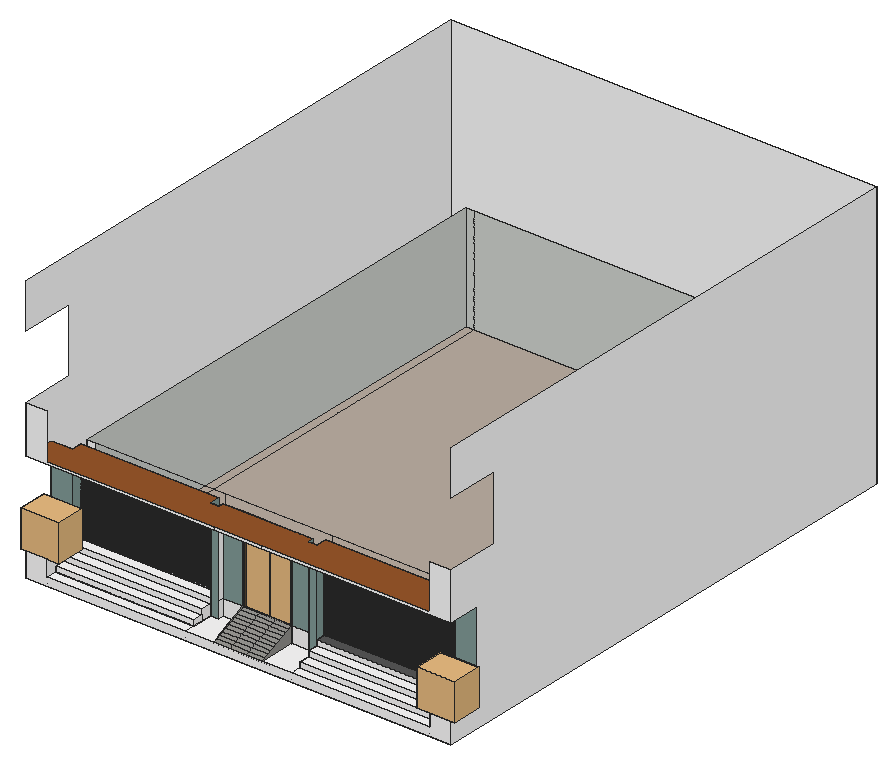
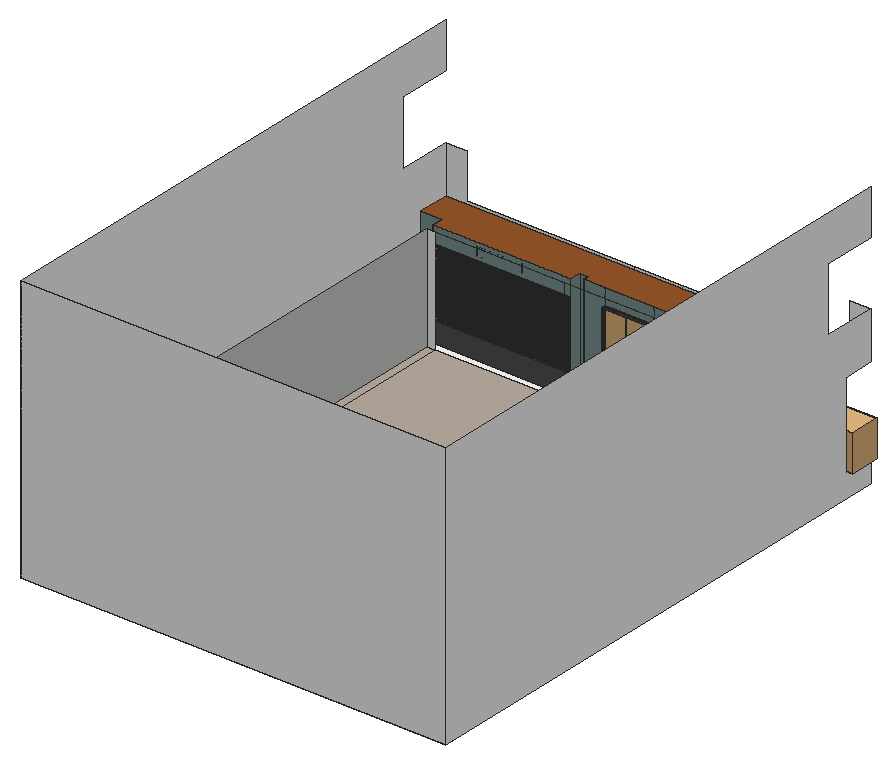
# SketchUp Ruby script. Lengths in inches.
U = 1.inch
M = Sketchup.active_model
def pt(a) = Geom::Point3d.new(a.map { |v| v * U })
def face(e, loops, mat)
  f = e.add_face(loops[0].map { |a| pt(a) })
  loops[1..].each { |l| e.add_face(l.map { |a| pt(a) }).erase! }
  f.material = f.back_material = mat if mat
  f
end
# faces: each face lists its corners as indices into pts; further lists are holes
def faces(e, pts, list, mat = nil) = list.each { |f| face(e, (f[0].is_a?(Array) ? f : [f]).map { |l| l.map { |i| pts[i] } }, mat) }
# xy, xz, yz: faces in a plane at the given z, y or x. An outline is a flat list of corners, or four numbers for a rectangle; further outlines are holes
def ring(l) = l.size == 4 ? [[l[0], l[1]], [l[2], l[1]], [l[2], l[3]], [l[0], l[3]]] : l.each_slice(2).to_a
def flat(e, list, mat, &to3) = list.each { |f| face(e, (f[0].is_a?(Array) ? f : [f]).map { |l| ring(l).map { |u, v| to3.(u, v) } }, mat) }
def xy(e, z, list, mat = nil) = flat(e, list, mat) { |x, y| [x, y, z] }
def xz(e, y, list, mat = nil) = flat(e, list, mat) { |x, z| [x, y, z] }
def yz(e, x, list, mat = nil) = flat(e, list, mat) { |y, z| [x, y, z] }
def lines(e, pts, list) = list.each { |a, b| e.add_line(pt(pts[a]), pt(pts[b])) }
# prism: a flat outline (further loops are holes) pulled along v
def prism(e, loops, v, mat = nil)
  f = face(e, loops, mat); d = Geom::Vector3d.new(v.map { |x| x * U })
  f.pushpull(f.normal.samedirection?(d) ? d.length : -d.length)
end
def box(e, o, s, mat = nil) = prism(e, [[o, [o[0] + s[0], o[1], o[2]], [o[0] + s[0], o[1] + s[1], o[2]], [o[0], o[1] + s[1], o[2]]]], [0, 0, s[2]], mat)
def at(x, y, z, deg = 0) = Geom::Transformation.translation(pt([x, y, z])) * Geom::Transformation.rotation(ORIGIN, Z_AXIS, deg.degrees)
def axes(o, x, y, z) = Geom::Transformation.new([*x, 0, *y, 0, *z, 0, *pt(o).to_a, 1])
def part(name) = M.definitions.add(name)
# library, detail: a bought-in or finely detailed component or shape, given as its bounding box
def library(name, o, s) = part(name).tap { |d| box(d.entities, o, s) }
def detail(e, o, s) = box(e.add_group.entities, o, s)
def put(e, d, t, mat = nil) = e.add_instance(d, t).tap { |i| i.material = mat if mat }
def group(e, t, mat = nil) = e.add_group.tap { |g| g.transformation = t; g.material = mat if mat }.entities
root = M.entities
M.materials.add("LAM 2").color = [91, 74, 54]
M.materials.add("LAM 2\#1").color = [121, 98, 72]
M.materials.add("W144X970F75_NILAYA EQUINOX FD25757 ROLL F75").color = [139, 163, 155]
M.materials.add("W144X977F75_NILAYA EQUINOX FD25283 ROLL F75").color = [131, 158, 154]
M.materials.add("W146Z451B75_NILAYA CITY GLAM 32602 ROLL B75").color = [212, 216, 211]
M.materials.add("YELLOW V").color = [99, 70, 40]
M.materials.add("[0135_DarkGray]").color = [81, 81, 81]
M.materials.add("[Color L01]1").color = [255, 254, 254]
M.materials.add("[Color M00]").color = [255, 255, 255]
M.materials.add("[Color M06]").color = [86, 86, 86]
M.materials.add("[Encaustic Tile Circular 02]").color = [187, 174, 162]
M.materials.add("[Granite Light Gray]").color = [149, 148, 144]
M.materials.add("[Metal Silver]").color = [234, 233, 238]
M.materials.add("[Translucent Glass Gray]").color = [128, 128, 128]
M.materials["[Translucent Glass Gray]"].alpha = 0.5
M.materials.add("[Wood Cherry Original]").color = [152, 86, 42]
c1 = part("Group\#11")
p = [[0,5.39,1.97],[-0.2,123.5,1.97],[-0.2,123.5,0],[0,5.39,0],[0,5.39,0.39]]
faces(c1.entities,p,[[0,1,2,3,4]],"[Metal Silver]")
c2 = part("Group\#41")
g1 = group(c2.entities,at(58.46,4.92,0,180),"YELLOW V")
xy(g1,0,[[0,0,0,4.92,1.5,4.92,1.5,3.35,1.97,3.35,1.97,0]])
xy(g1,82.2,[[1.97,0,15.59,3.35]])
xy(g1,82.68,[[1.5,3.35,15.59,4.92]])
xy(g1,84.17,[[0,0,15.59,4.92]])
xz(g1,0,[[0,0,1.97,0,1.97,82.2,15.59,82.2,15.59,84.17,0,84.17]])
xz(g1,3.35,[[1.5,0,1.5,82.68,15.59,82.68,15.59,82.2,1.97,82.2,1.97,0]])
xz(g1,4.92,[[0,0,0,84.17,1.5,82.68,1.5,0]],"LAM 2")
xz(g1,4.92,[[1.5,82.68,0,84.17,15.59,84.17,15.59,82.68]],"LAM 2\#1")
yz(g1,0,[[0,0,4.92,84.17]])
yz(g1,1.5,[[3.35,0,4.92,82.68]])
yz(g1,1.97,[[0,0,3.35,82.2]])
yz(g1,15.59,[[0,82.2,3.35,82.2,3.35,82.68,4.92,82.68,4.92,84.17,0,84.17]])
g2 = group(c2.entities,at(0.47,4.92,0),"LAM 2")
xy(g2,0,[[0,-4.92,1.5,-4.92,1.5,-3.35,1.97,-3.35,1.97,0,0,0]])
xy(g2,82.2,[[1.97,-3.35,50.39,0]])
xy(g2,82.68,[[1.5,-4.92,50.39,-3.35]])
xy(g2,84.17,[[0,-4.92,50.39,0]])
xz(g2,-4.92,[[0,0,0,84.17,1.5,82.68,1.5,0]],"LAM 2")
xz(g2,-4.92,[[1.5,82.68,0,84.17,50.39,84.17,50.39,82.68]],"LAM 2\#1")
xz(g2,-3.35,[[1.5,0,1.5,82.68,50.39,82.68,50.39,82.2,1.97,82.2,1.97,0]])
xz(g2,0,[[0,0,1.97,0,1.97,82.2,50.39,82.2,50.39,84.17,0,84.17]])
yz(g2,0,[[-4.92,0,0,84.17]])
yz(g2,1.5,[[-4.92,0,-3.35,82.68]])
yz(g2,1.97,[[-3.35,0,0,82.2]])
yz(g2,50.39,[[-3.35,82.2,-3.35,82.68,-4.92,82.68,-4.92,84.17,0,84.17,0,82.2]])
c3 = part("Component\#1")
xy(c3.entities,-3.54,[[0,0,0.625,1.97]],"[Metal Silver]")
xy(c3.entities,98.82,[[0,0,0.33,1.97],[0.33,0,0.625,1.97]],"[Metal Silver]")
xz(c3.entities,0,[[0,-3.54,0.625,98.82]],"[Metal Silver]")
xz(c3.entities,1.97,[[0,-3.54,0.625,98.82]],"[Metal Silver]")
yz(c3.entities,0,[[0,-3.54,1.97,98.82]],"[Metal Silver]")
yz(c3.entities,0.625,[[0,-3.54,1.97,98.82]],"[Metal Silver]")
p = [[0.2,1.91,87.01],[0.2,1.97,87.01],[0,1.97,-3.15],[0.2,1.97,-3.15]]
lines(c3.entities,p,[[0,1],[2,3]])
c4 = library("0ed0d9b5-8e27-4f25-b4f0-a8b44624208f",[-19.74,-16.15,0],[43.07,33.13,41.46])
c5 = library("Group\#72",[0,0,0],[27.68,2.95,82.68])
c6 = part("Component\#10")
p = [[0,5.45,0],[0,123.5625,0],[0.07,123.5625,0.15],[0.07,5.45,0.15],[0.13,123.5625,0.3125],[0.13,5.45,0.3125],
  [0.18,123.5625,0.48],[0.18,5.45,0.48],[0.21,123.5625,0.65],[0.21,5.45,0.65],[0.23,123.5625,0.8125],[0.23,5.45,0.8125],
  [0.24,123.5625,0.98],[0.24,5.45,0.98],[0.23,123.5625,1.15],[0.23,5.45,1.15],[0.21,123.5625,1.32],[0.21,5.45,1.32],
  [0.18,123.5625,1.49],[0.18,5.45,1.49],[0.13,123.5625,1.65],[0.13,5.45,1.65],[0.07,123.5625,1.8125],[0.07,5.45,1.8125],
  [0,123.5625,1.97],[0,5.45,1.97]]
faces(c6.entities,p,[[0,1,2,3],[3,2,4,5],[5,4,6,7],[7,6,8,9],[9,8,10,11],[11,10,12,13],[13,12,14,15],[15,14,16,17],
  [17,16,18,19],[19,18,20,21],[21,20,22,23],[23,22,24,25]],"[Metal Silver]")
c7 = part("Group\#70")
prism(c7.entities,[[[-3.9375,3.9375,0.03],[-3.9375,2.11,0.45],[-3.9375,0.7,1.7],[-3.9375,0.03,3.46],[-3.9375,0.26,5.33],[-3.9375,1.33,6.88],[-3.9375,2.99,7.76],[-3.9375,4.88,7.76],[-3.9375,6.55,6.88],[-3.9375,7.62,5.33],[-3.9375,7.85,3.46],[-3.9375,7.18,1.7],[-3.9375,5.77,0.45]]],[118.11,0,0],"[Metal Silver]")
p = [[-3.9375,3.9375,0.03],[-3.9375,3.9375,0]]
lines(c7.entities,p,[[0,1]])
c8 = library("SHOP-2\#1",[0.4375,0,0],[50.6875,9.31,3])
c9 = library("SHOP-1",[0.4375,0,0],[49.04,9.31,3])
xy(root,-3,[[0,0,480,600]],"[Color M00]")
xy(root,0,[[24,12,180,48],[300,12,456,48]],"[Color M06]")
xy(root,0,[[24,57,33,591],[33,57,447,591],[447,57,456,591]],"[Encaustic Tile Circular 02]")
xy(root,6,[[24,0,180,12],[180,0,211.83,0,211.83,42,189,42,189,36,180,36],[267,0,300,0,300,36,291,36,291,42,267,42],[300,0,456,12]],"[Color L01]1")
xy(root,6,[[211.83,0,267,42]],"[Granite Light Gray]")
xy(root,12,[[24,12,180,24],[300,12,456,24]],"[Color L01]1")
xy(root,18,[[24,24,180,36],[300,24,456,36]],"[Color L01]1")
xy(root,24,[[0,0,24,36],[456,0,480,36],[24,36,180,48],[211.83,42,267,57]],"[Color L01]1")
xy(root,24,[[300,36,456,48]],"[Color M06]")
xy(root,120,[[0,0,0,36,24,36,24,48,180,48,180,36,189,36,189,42,291,42,291,36,300,36,300,48,456,48,456,36,480,36,480,0]],"[Wood Cherry Original]")
xz(root,0,[[0,-3,480,-3,480,24,456,24,456,6,24,6,24,24,0,24]],"[Color L01]1")
xz(root,0,[[0,120,211.83,120,211.83,123,24,123,24,174.0625,0,174.0625],[211.83,120,267,123],[267,120,480,120,480,173.5625,456,173.5625,456,123,267,123]],"[Color M00]")
xz(root,12,[[24,6,180,12],[300,6,456,12]],"[Color L01]1")
xz(root,12,[[24,0,180,6]],"[Color M06]")
xz(root,24,[[24,12,180,18],[300,12,456,18]],"[Color L01]1")
xz(root,36,[[180,6,189,120],[291,6,300,120],[0,24,24,120],[456,24,480,120]],"W144X977F75_NILAYA EQUINOX FD25283 ROLL F75")
xz(root,36,[[24,18,180,24],[300,18,456,24]],"[Color L01]1")
xz(root,42,[[189,24,211.83,120],[267,24,291,120],[211.83,102,267,120]],"W144X977F75_NILAYA EQUINOX FD25283 ROLL F75")
xz(root,42,[[189,6,211.83,24],[211.83,6,267,24],[267,6,291,24]],"[Color L01]1")
xz(root,48,[[24,102,180,120],[300,102,456,120]],"W144X977F75_NILAYA EQUINOX FD25283 ROLL F75")
xz(root,48,[[24,0,180,24],[300,0,456,24]],"[Color M06]")
xz(root,57,[[211.83,0,267,24]],"[Color L01]1")
xz(root,57,[[24,0,33,120],[447,0,456,120]],"[Color M00]")
xz(root,591,[[24,0,33,120],[33,0,447,120],[447,0,456,120]],"W146Z451B75_NILAYA CITY GLAM 32602 ROLL B75")
xz(root,600,[[0,-3,480,297.0625]],"[Color M00]")
yz(root,0,[[0,-3,0,24,36,24,36,120,0,120,0,174.0625,60.9375,174.0625,60.9375,246.0625,0,246.0625,0,297.0625,600,297.0625,600,-3]],"[Color M00]")
yz(root,24,[[36,24,48,120]],"W144X977F75_NILAYA EQUINOX FD25283 ROLL F75")
yz(root,24,[[57,0,591,120]],"W146Z451B75_NILAYA CITY GLAM 32602 ROLL B75")
yz(root,24,[[0,6,12,6,12,12,24,12,24,18,36,18,36,24,0,24]],"[Color L01]1")
yz(root,24,[[12,0,48,0,48,24,36,24,36,18,24,18,24,12,12,12]],"[Color M06]")
yz(root,180,[[36,24,48,120]],"W144X977F75_NILAYA EQUINOX FD25283 ROLL F75")
yz(root,180,[[12,0,36,6],[12,6,24,12],[24,6,36,18]],"[Color L01]1")
yz(root,180,[[36,0,48,24]],"[Color M06]")
yz(root,189,[[36,6,42,24],[36,24,42,120]],"[Color L01]1")
yz(root,211.83,[[42,0,57,24],[0,6,42,24,42,6]],"[Granite Light Gray]")
yz(root,267,[[42,0,57,24],[0,6,42,6,42,24]],"[Granite Light Gray]")
yz(root,291,[[36,24,42,120]],"W144X977F75_NILAYA EQUINOX FD25283 ROLL F75")
yz(root,291,[[36,6,42,24]],"[Color L01]1")
yz(root,300,[[36,24,48,120]],"W144X977F75_NILAYA EQUINOX FD25283 ROLL F75")
yz(root,300,[[12,0,36,6],[12,6,24,12],[24,6,36,18]],"[Color L01]1")
yz(root,300,[[36,0,48,24]],"[Color M06]")
yz(root,456,[[36,24,48,120]],"W144X977F75_NILAYA EQUINOX FD25283 ROLL F75")
yz(root,456,[[57,0,591,120]],"W146Z451B75_NILAYA CITY GLAM 32602 ROLL B75")
yz(root,456,[[0,6,0,24,36,24,36,18,24,18,24,12,12,12,12,6]],"[Color L01]1")
yz(root,456,[[12,0,48,0,48,24,36,24,36,18,24,18,24,12,12,12]],"[Color M06]")
yz(root,480,[[0,-3,600,-3,600,297.0625,0,297.0625,0,246.0625,60.3125,246.0625,60.3125,174.0625,60,174.0625,60,173.5625,0,173.5625,0,120,36,120,36,24,0,24]],"[Color M00]")
p = [[230.22,0,6],[230.22,4.2,7.8],[211.83,4.2,7.8],[211.83,0,6],[248.61,0,6],[248.61,4.2,7.8],
  [267,0,6],[267,4.2,7.8],[230.22,8.4,9.6],[211.83,8.4,9.6],[248.61,8.4,9.6],[267,8.4,9.6],
  [230.22,12.6,11.4],[211.83,12.6,11.4],[248.61,12.6,11.4],[267,12.6,11.4],[230.22,16.8,13.2],[211.83,16.8,13.2],
  [248.61,16.8,13.2],[267,16.8,13.2],[230.22,21,15],[211.83,21,15],[248.61,21,15],[267,21,15],
  [230.22,25.2,16.8],[211.83,25.2,16.8],[248.61,25.2,16.8],[267,25.2,16.8],[230.22,29.4,18.6],[211.83,29.4,18.6],
  [248.61,29.4,18.6],[267,29.4,18.6],[230.22,33.6,20.4],[211.83,33.6,20.4],[248.61,33.6,20.4],[267,33.6,20.4],
  [230.22,37.8,22.2],[211.83,37.8,22.2],[248.61,37.8,22.2],[267,37.8,22.2],[211.83,42,24],[230.22,42,24],
  [248.61,42,24],[267,42,24],[24,0,0],[24,12,0],[180,0,0],[180,12,0],
  [456,0,0],[456,12,0],[300,0,0],[300,12,0],[456,24,2.25],[300,24,2.25],
  [456,12,2.25],[300,12,2.25],[300,57,120],[447,57,120],[180,57,120],[33,57,120],
  [300,57,0],[180,57,0],[31.55,48.43,98.99],[172.28,48.43,98.99],[307.55,46.28,98.99],[448.28,46.28,98.99]]
faces(root,p,[[0,1,2,3],[4,5,1,0],[6,7,5,4],[1,8,9,2],[5,10,8,1],[7,11,10,5],[8,12,13,9],[10,14,12,8],
  [11,15,14,10],[12,16,17,13],[14,18,16,12],[15,19,18,14],[16,20,21,17],[18,22,20,16],[19,23,22,18],[20,24,25,21],
  [22,26,24,20],[23,27,26,22],[24,28,29,25],[26,30,28,24],[27,31,30,26],[28,32,33,29],[30,34,32,28],[31,35,34,30],
  [32,36,37,33],[34,38,36,32],[35,39,38,34],[40,37,36,41],[41,36,38,42],[42,38,39,43]],"[Granite Light Gray]")
lines(root,p,[[44,45],[46,47],[48,49],[50,51],[52,53],[54,55],[56,57],[58,56],[59,58],[60,56],[61,58],[62,63],
  [64,65]])
put(root,c1,axes([19.625,48.43,24],[0,-1,0],[1.27819,0,0],[0,0,0.7326]),"[Translucent Glass Gray]")
put(root,c1,axes([295.625,46.28,24],[0,-1,0],[1.27819,0,0],[0,0,0.7326]),"[Translucent Glass Gray]")
put(root,c2,axes([211.38,44.81,24],[0.95143,0,0],[0,-0.57,0],[0,0,0.92666]),"LAM 2")
put(root,c3,axes([177.48,48.625,26.6],[0,-1,0],[1.27819,0,0],[0,0,0.7326]),"W144X977F75_NILAYA EQUINOX FD25283 ROLL F75")
put(root,c4,at(13.74,16.15,24))
put(root,c4,at(465.21,11.53,24))
put(root,c3,axes([24,48.625,26.6],[0,-1,0],[1.27819,0,0],[0,0,0.7326]),"[0135_DarkGray]")
put(root,c5,axes([213.125,43.01,24],[1,0,0],[0,0.57,0],[0,0,0.92666]))
put(root,c5,axes([268.45,43.01,24],[-1,0,0],[0,0.57,0],[0,0,0.92666]))
put(root,c3,axes([453.48,46.47,26.6],[0,-1,0],[1.27819,0,0],[0,0,0.7326]),"[0135_DarkGray]")
put(root,c3,axes([300,46.47,26.6],[0,-1,0],[1.27819,0,0],[0,0,0.7326]),"[0135_DarkGray]")
put(root,c6,axes([19.54,48.43,25.44],[0,-1,0],[1.27819,0,0],[0,0,0.7326]),"[Translucent Glass Gray]")
put(root,c6,axes([295.54,46.28,25.44],[0,-1,0],[1.27819,0,0],[0,0,0.7326]),"[Translucent Glass Gray]")
put(root,c6,axes([19.54,48.43,26.88],[0,-1,0],[1.27819,0,0],[0,0,0.7326]),"[Translucent Glass Gray]")
put(root,c6,axes([295.54,46.28,26.88],[0,-1,0],[1.27819,0,0],[0,0,0.7326]),"[Translucent Glass Gray]")
put(root,c6,axes([19.54,48.43,28.33],[0,-1,0],[1.27819,0,0],[0,0,0.7326]),"[Translucent Glass Gray]")
put(root,c6,axes([295.54,46.28,28.33],[0,-1,0],[1.27819,0,0],[0,0,0.7326]),"[Translucent Glass Gray]")
put(root,c6,axes([19.54,48.43,29.77],[0,-1,0],[1.27819,0,0],[0,0,0.7326]),"[Translucent Glass Gray]")
put(root,c6,axes([295.54,46.28,29.77],[0,-1,0],[1.27819,0,0],[0,0,0.7326]),"[Translucent Glass Gray]")
put(root,c6,axes([19.54,48.43,31.21],[0,-1,0],[1.27819,0,0],[0,0,0.7326]),"[Translucent Glass Gray]")
put(root,c6,axes([295.54,46.28,31.21],[0,-1,0],[1.27819,0,0],[0,0,0.7326]),"[Translucent Glass Gray]")
put(root,c6,axes([19.54,48.43,32.65],[0,-1,0],[1.27819,0,0],[0,0,0.7326]),"[Translucent Glass Gray]")
put(root,c6,axes([295.54,46.28,32.65],[0,-1,0],[1.27819,0,0],[0,0,0.7326]),"[Translucent Glass Gray]")
put(root,c6,axes([19.54,48.43,34.09],[0,-1,0],[1.27819,0,0],[0,0,0.7326]),"[Translucent Glass Gray]")
put(root,c6,axes([295.54,46.28,34.09],[0,-1,0],[1.27819,0,0],[0,0,0.7326]),"[Translucent Glass Gray]")
put(root,c6,axes([19.54,48.43,35.54],[0,-1,0],[1.27819,0,0],[0,0,0.7326]),"[Translucent Glass Gray]")
put(root,c6,axes([295.54,46.28,35.54],[0,-1,0],[1.27819,0,0],[0,0,0.7326]),"[Translucent Glass Gray]")
put(root,c6,axes([19.54,48.43,36.98],[0,-1,0],[1.27819,0,0],[0,0,0.7326]),"[Translucent Glass Gray]")
put(root,c6,axes([295.54,46.28,36.98],[0,-1,0],[1.27819,0,0],[0,0,0.7326]),"[Translucent Glass Gray]")
put(root,c6,axes([19.54,48.43,38.42],[0,-1,0],[1.27819,0,0],[0,0,0.7326]),"[Translucent Glass Gray]")
put(root,c6,axes([295.54,46.28,38.42],[0,-1,0],[1.27819,0,0],[0,0,0.7326]),"[Translucent Glass Gray]")
put(root,c6,axes([19.54,48.43,39.86],[0,-1,0],[1.27819,0,0],[0,0,0.7326]),"[Translucent Glass Gray]")
put(root,c6,axes([295.54,46.28,39.86],[0,-1,0],[1.27819,0,0],[0,0,0.7326]),"[Translucent Glass Gray]")
put(root,c6,axes([19.54,48.43,41.31],[0,-1,0],[1.27819,0,0],[0,0,0.7326]),"[Translucent Glass Gray]")
put(root,c6,axes([295.54,46.28,41.31],[0,-1,0],[1.27819,0,0],[0,0,0.7326]),"[Translucent Glass Gray]")
put(root,c6,axes([19.54,48.43,42.75],[0,-1,0],[1.27819,0,0],[0,0,0.7326]),"[Translucent Glass Gray]")
put(root,c6,axes([295.54,46.28,42.75],[0,-1,0],[1.27819,0,0],[0,0,0.7326]),"[Translucent Glass Gray]")
put(root,c6,axes([19.54,48.43,44.19],[0,-1,0],[1.27819,0,0],[0,0,0.7326]),"[Translucent Glass Gray]")
put(root,c6,axes([295.54,46.28,44.19],[0,-1,0],[1.27819,0,0],[0,0,0.7326]),"[Translucent Glass Gray]")
put(root,c6,axes([19.54,48.43,45.63],[0,-1,0],[1.27819,0,0],[0,0,0.7326]),"[Translucent Glass Gray]")
put(root,c6,axes([295.54,46.28,45.63],[0,-1,0],[1.27819,0,0],[0,0,0.7326]),"[Translucent Glass Gray]")
put(root,c6,axes([19.54,48.43,47.07],[0,-1,0],[1.27819,0,0],[0,0,0.7326]),"[Translucent Glass Gray]")
put(root,c6,axes([295.54,46.28,47.07],[0,-1,0],[1.27819,0,0],[0,0,0.7326]),"[Translucent Glass Gray]")
put(root,c6,axes([19.54,48.43,48.52],[0,-1,0],[1.27819,0,0],[0,0,0.7326]),"[Translucent Glass Gray]")
put(root,c6,axes([295.54,46.28,48.52],[0,-1,0],[1.27819,0,0],[0,0,0.7326]),"[Translucent Glass Gray]")
put(root,c6,axes([19.54,48.43,49.96],[0,-1,0],[1.27819,0,0],[0,0,0.7326]),"[Translucent Glass Gray]")
put(root,c6,axes([295.54,46.28,49.96],[0,-1,0],[1.27819,0,0],[0,0,0.7326]),"[Translucent Glass Gray]")
put(root,c6,axes([19.54,48.43,51.4],[0,-1,0],[1.27819,0,0],[0,0,0.7326]),"[Translucent Glass Gray]")
put(root,c6,axes([295.54,46.28,51.4],[0,-1,0],[1.27819,0,0],[0,0,0.7326]),"[Translucent Glass Gray]")
put(root,c6,axes([19.54,48.43,52.84],[0,-1,0],[1.27819,0,0],[0,0,0.7326]),"[Translucent Glass Gray]")
put(root,c6,axes([295.54,46.28,52.84],[0,-1,0],[1.27819,0,0],[0,0,0.7326]),"[Translucent Glass Gray]")
put(root,c6,axes([19.54,48.43,54.28],[0,-1,0],[1.27819,0,0],[0,0,0.7326]),"[Translucent Glass Gray]")
put(root,c6,axes([295.54,46.28,54.28],[0,-1,0],[1.27819,0,0],[0,0,0.7326]),"[Translucent Glass Gray]")
put(root,c6,axes([19.54,48.43,55.73],[0,-1,0],[1.27819,0,0],[0,0,0.7326]),"[Translucent Glass Gray]")
put(root,c6,axes([295.54,46.28,55.73],[0,-1,0],[1.27819,0,0],[0,0,0.7326]),"[Translucent Glass Gray]")
put(root,c6,axes([19.54,48.43,57.17],[0,-1,0],[1.27819,0,0],[0,0,0.7326]),"[Translucent Glass Gray]")
put(root,c6,axes([295.54,46.28,57.17],[0,-1,0],[1.27819,0,0],[0,0,0.7326]),"[Translucent Glass Gray]")
put(root,c6,axes([19.54,48.43,58.61],[0,-1,0],[1.27819,0,0],[0,0,0.7326]),"[Translucent Glass Gray]")
put(root,c6,axes([295.54,46.28,58.61],[0,-1,0],[1.27819,0,0],[0,0,0.7326]),"[Translucent Glass Gray]")
put(root,c6,axes([19.54,48.43,60.05],[0,-1,0],[1.27819,0,0],[0,0,0.7326]),"[Translucent Glass Gray]")
put(root,c6,axes([295.54,46.28,60.05],[0,-1,0],[1.27819,0,0],[0,0,0.7326]),"[Translucent Glass Gray]")
put(root,c6,axes([19.54,48.43,61.5],[0,-1,0],[1.27819,0,0],[0,0,0.7326]),"[Translucent Glass Gray]")
put(root,c6,axes([295.54,46.28,61.5],[0,-1,0],[1.27819,0,0],[0,0,0.7326]),"[Translucent Glass Gray]")
put(root,c6,axes([19.54,48.43,62.9375],[0,-1,0],[1.27819,0,0],[0,0,0.7326]),"[Translucent Glass Gray]")
put(root,c6,axes([295.54,46.28,62.9375],[0,-1,0],[1.27819,0,0],[0,0,0.7326]),"[Translucent Glass Gray]")
put(root,c6,axes([19.54,48.43,64.38],[0,-1,0],[1.27819,0,0],[0,0,0.7326]),"[Translucent Glass Gray]")
put(root,c6,axes([295.54,46.28,64.38],[0,-1,0],[1.27819,0,0],[0,0,0.7326]),"[Translucent Glass Gray]")
put(root,c6,axes([19.54,48.43,65.82],[0,-1,0],[1.27819,0,0],[0,0,0.7326]),"[Translucent Glass Gray]")
put(root,c6,axes([295.54,46.28,65.82],[0,-1,0],[1.27819,0,0],[0,0,0.7326]),"[Translucent Glass Gray]")
put(root,c6,axes([19.54,48.43,67.26],[0,-1,0],[1.27819,0,0],[0,0,0.7326]),"[Translucent Glass Gray]")
put(root,c6,axes([295.54,46.28,67.26],[0,-1,0],[1.27819,0,0],[0,0,0.7326]),"[Translucent Glass Gray]")
put(root,c6,axes([19.54,48.43,68.71],[0,-1,0],[1.27819,0,0],[0,0,0.7326]),"[Translucent Glass Gray]")
put(root,c6,axes([295.54,46.28,68.71],[0,-1,0],[1.27819,0,0],[0,0,0.7326]),"W144X970F75_NILAYA EQUINOX FD25757 ROLL F75")
put(root,c6,axes([19.54,48.43,70.15],[0,-1,0],[1.27819,0,0],[0,0,0.7326]),"[Translucent Glass Gray]")
put(root,c6,axes([295.54,46.28,70.15],[0,-1,0],[1.27819,0,0],[0,0,0.7326]),"[Translucent Glass Gray]")
put(root,c6,axes([19.54,48.43,71.59],[0,-1,0],[1.27819,0,0],[0,0,0.7326]),"[Translucent Glass Gray]")
put(root,c6,axes([295.54,46.28,71.59],[0,-1,0],[1.27819,0,0],[0,0,0.7326]),"[Translucent Glass Gray]")
put(root,c6,axes([19.54,48.43,73.03],[0,-1,0],[1.27819,0,0],[0,0,0.7326]),"[Translucent Glass Gray]")
put(root,c6,axes([295.54,46.28,73.03],[0,-1,0],[1.27819,0,0],[0,0,0.7326]),"[Translucent Glass Gray]")
put(root,c6,axes([19.54,48.43,74.47],[0,-1,0],[1.27819,0,0],[0,0,0.7326]),"[Translucent Glass Gray]")
put(root,c6,axes([295.54,46.28,74.47],[0,-1,0],[1.27819,0,0],[0,0,0.7326]),"[Translucent Glass Gray]")
put(root,c6,axes([19.54,48.43,75.92],[0,-1,0],[1.27819,0,0],[0,0,0.7326]),"[Translucent Glass Gray]")
put(root,c6,axes([295.54,46.28,75.92],[0,-1,0],[1.27819,0,0],[0,0,0.7326]),"[Translucent Glass Gray]")
put(root,c6,axes([19.54,48.43,77.36],[0,-1,0],[1.27819,0,0],[0,0,0.7326]),"[Translucent Glass Gray]")
put(root,c6,axes([295.54,46.28,77.36],[0,-1,0],[1.27819,0,0],[0,0,0.7326]),"[Translucent Glass Gray]")
put(root,c6,axes([19.54,48.43,78.8],[0,-1,0],[1.27819,0,0],[0,0,0.7326]),"[Translucent Glass Gray]")
put(root,c6,axes([295.54,46.28,78.8],[0,-1,0],[1.27819,0,0],[0,0,0.7326]),"[Translucent Glass Gray]")
put(root,c6,axes([19.54,48.43,80.24],[0,-1,0],[1.27819,0,0],[0,0,0.7326]),"[Translucent Glass Gray]")
put(root,c6,axes([295.54,46.28,80.24],[0,-1,0],[1.27819,0,0],[0,0,0.7326]),"[Translucent Glass Gray]")
put(root,c6,axes([19.54,48.43,81.69],[0,-1,0],[1.27819,0,0],[0,0,0.7326]),"[Translucent Glass Gray]")
put(root,c6,axes([295.54,46.28,81.69],[0,-1,0],[1.27819,0,0],[0,0,0.7326]),"[Translucent Glass Gray]")
put(root,c6,axes([19.54,48.43,83.13],[0,-1,0],[1.27819,0,0],[0,0,0.7326]),"[Translucent Glass Gray]")
put(root,c6,axes([295.54,46.28,83.13],[0,-1,0],[1.27819,0,0],[0,0,0.7326]),"[Translucent Glass Gray]")
put(root,c6,axes([19.54,48.43,84.57],[0,-1,0],[1.27819,0,0],[0,0,0.7326]),"[Translucent Glass Gray]")
put(root,c6,axes([295.54,46.28,84.57],[0,-1,0],[1.27819,0,0],[0,0,0.7326]),"[Translucent Glass Gray]")
put(root,c6,axes([19.54,48.43,86.01],[0,-1,0],[1.27819,0,0],[0,0,0.7326]),"[Translucent Glass Gray]")
put(root,c6,axes([295.54,46.28,86.01],[0,-1,0],[1.27819,0,0],[0,0,0.7326]),"[Translucent Glass Gray]")
put(root,c6,axes([19.54,48.43,87.45],[0,-1,0],[1.27819,0,0],[0,0,0.7326]),"[Translucent Glass Gray]")
put(root,c6,axes([295.54,46.28,87.45],[0,-1,0],[1.27819,0,0],[0,0,0.7326]),"[Translucent Glass Gray]")
put(root,c6,axes([19.54,48.43,88.9],[0,-1,0],[1.27819,0,0],[0,0,0.7326]),"[Translucent Glass Gray]")
put(root,c6,axes([295.54,46.28,88.9],[0,-1,0],[1.27819,0,0],[0,0,0.7326]),"[Translucent Glass Gray]")
put(root,c6,axes([19.54,48.43,90.34],[0,-1,0],[1.27819,0,0],[0,0,0.7326]),"[Translucent Glass Gray]")
put(root,c6,axes([295.54,46.28,90.34],[0,-1,0],[1.27819,0,0],[0,0,0.7326]),"[Translucent Glass Gray]")
put(root,c6,axes([19.54,48.43,91.78],[0,-1,0],[1.27819,0,0],[0,0,0.7326]),"[Translucent Glass Gray]")
put(root,c6,axes([295.54,46.28,91.78],[0,-1,0],[1.27819,0,0],[0,0,0.7326]),"[Translucent Glass Gray]")
put(root,c6,axes([19.54,48.43,93.22],[0,-1,0],[1.27819,0,0],[0,0,0.7326]),"[Translucent Glass Gray]")
put(root,c6,axes([295.54,46.28,93.22],[0,-1,0],[1.27819,0,0],[0,0,0.7326]),"[Translucent Glass Gray]")
put(root,c6,axes([19.54,48.43,94.66],[0,-1,0],[1.27819,0,0],[0,0,0.7326]),"[Translucent Glass Gray]")
put(root,c6,axes([295.54,46.28,94.66],[0,-1,0],[1.27819,0,0],[0,0,0.7326]),"[Translucent Glass Gray]")
put(root,c6,axes([19.54,48.43,96.11],[0,-1,0],[1.27819,0,0],[0,0,0.7326]),"[Translucent Glass Gray]")
put(root,c6,axes([295.54,46.28,96.11],[0,-1,0],[1.27819,0,0],[0,0,0.7326]),"[Translucent Glass Gray]")
put(root,c7,axes([31.55,40.27,96.35],[1.27819,0,0],[0,1.04,0],[0,0,0.7619]))
put(root,c7,axes([307.55,38.12,96.35],[1.27819,0,0],[0,1.04,0],[0,0,0.7619]),"W144X977F75_NILAYA EQUINOX FD25283 ROLL F75")
put(root,c6,axes([19.54,48.43,97.55],[0,-1,0],[1.27819,0,0],[0,0,0.7326]),"[Translucent Glass Gray]")
put(root,c6,axes([295.54,46.28,97.55],[0,-1,0],[1.27819,0,0],[0,0,0.7326]),"[Translucent Glass Gray]")
put(root,c8,axes([354.83,48,106.16],[1,0,0],[0,0,1],[0,-1,0]))
put(root,c9,axes([74.84,48,106.85],[1,0,0],[0,0,1],[0,-1,0]))
